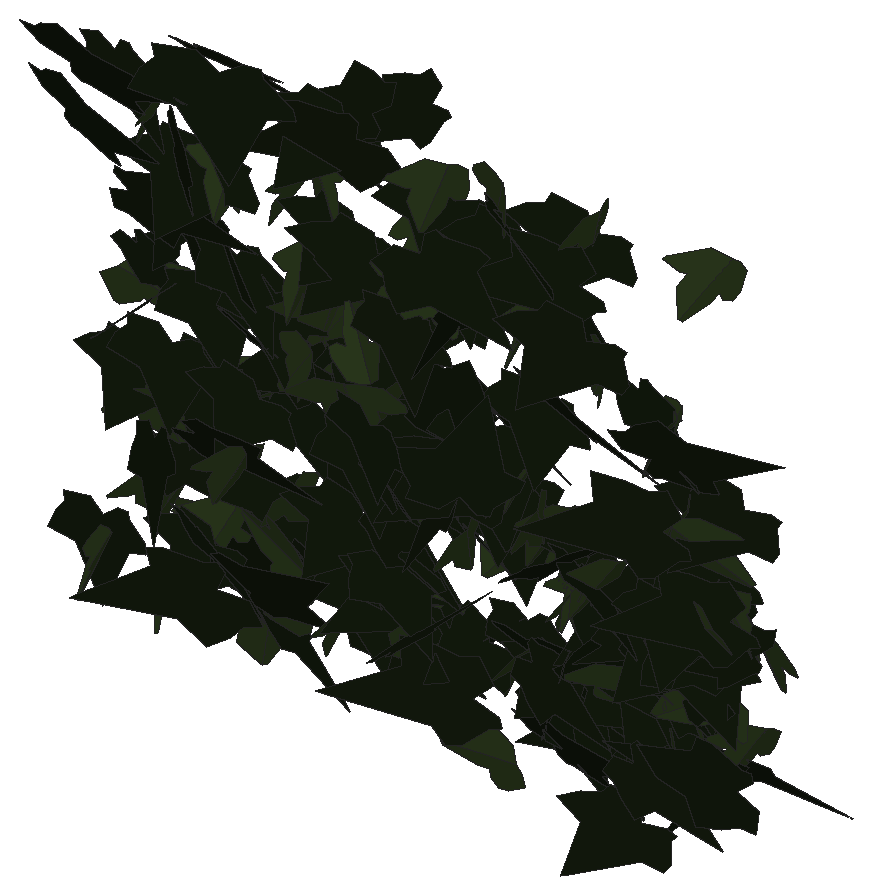
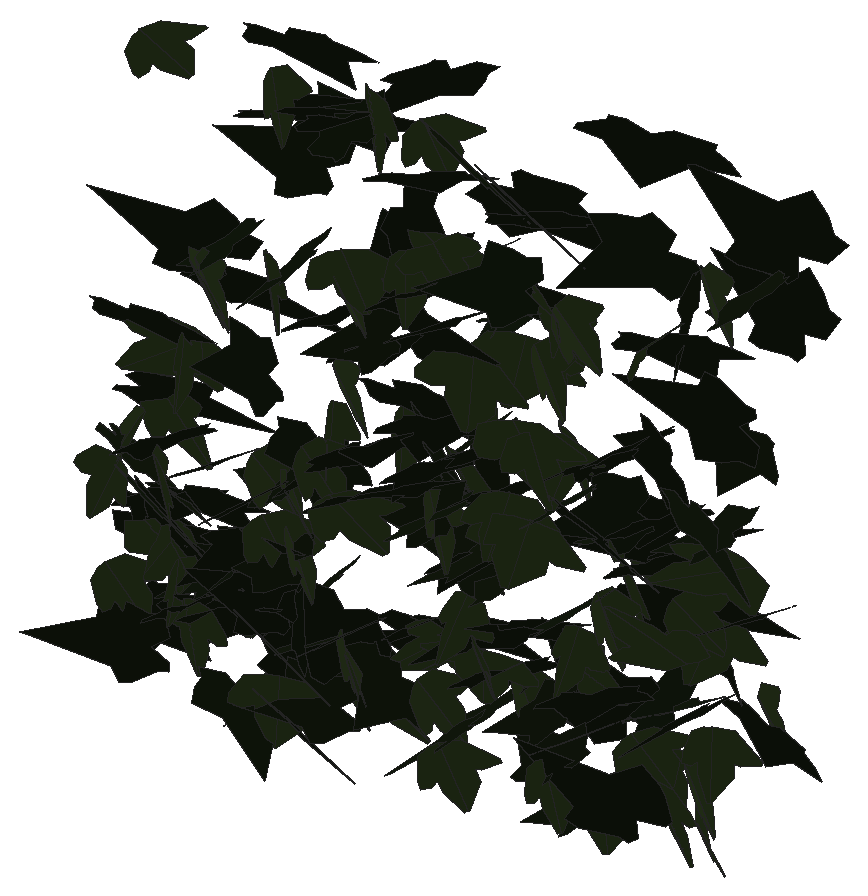
# SketchUp Ruby script. Lengths in millimetres.
U = 1.mm
M = Sketchup.active_model
def pt(a) = Geom::Point3d.new(a.map { |v| v * U })
def face(e, loops, mat)
  f = e.add_face(loops[0].map { |a| pt(a) })
  loops[1..].each { |l| e.add_face(l.map { |a| pt(a) }).erase! }
  f.material = f.back_material = mat if mat
  f
end
# faces: each face lists its corners as indices into pts; further lists are holes
def faces(e, pts, list, mat = nil) = list.each { |f| face(e, (f[0].is_a?(Array) ? f : [f]).map { |l| l.map { |i| pts[i] } }, mat) }
# xy, xz, yz: faces in a plane at the given z, y or x. An outline is a flat list of corners, or four numbers for a rectangle; further outlines are holes
def ring(l) = l.size == 4 ? [[l[0], l[1]], [l[2], l[1]], [l[2], l[3]], [l[0], l[3]]] : l.each_slice(2).to_a
def flat(e, list, mat, &to3) = list.each { |f| face(e, (f[0].is_a?(Array) ? f : [f]).map { |l| ring(l).map { |u, v| to3.(u, v) } }, mat) }
def xy(e, z, list, mat = nil) = flat(e, list, mat) { |x, y| [x, y, z] }
def xz(e, y, list, mat = nil) = flat(e, list, mat) { |x, z| [x, y, z] }
def yz(e, x, list, mat = nil) = flat(e, list, mat) { |y, z| [x, y, z] }
def lines(e, pts, list) = list.each { |a, b| e.add_line(pt(pts[a]), pt(pts[b])) }
# prism: a flat outline (further loops are holes) pulled along v
def prism(e, loops, v, mat = nil)
  f = face(e, loops, mat); d = Geom::Vector3d.new(v.map { |x| x * U })
  f.pushpull(f.normal.samedirection?(d) ? d.length : -d.length)
end
def box(e, o, s, mat = nil) = prism(e, [[o, [o[0] + s[0], o[1], o[2]], [o[0] + s[0], o[1] + s[1], o[2]], [o[0], o[1] + s[1], o[2]]]], [0, 0, s[2]], mat)
def at(x, y, z, deg = 0) = Geom::Transformation.translation(pt([x, y, z])) * Geom::Transformation.rotation(ORIGIN, Z_AXIS, deg.degrees)
def axes(o, x, y, z) = Geom::Transformation.new([*x, 0, *y, 0, *z, 0, *pt(o).to_a, 1])
def part(name) = M.definitions.add(name)
# library, detail: a bought-in or finely detailed component or shape, given as its bounding box
def library(name, o, s) = part(name).tap { |d| box(d.entities, o, s) }
def detail(e, o, s) = box(e.add_group.entities, o, s)
def put(e, d, t, mat = nil) = e.add_instance(d, t).tap { |i| i.material = mat if mat }
def group(e, t, mat = nil) = e.add_group.tap { |g| g.transformation = t; g.material = mat if mat }.entities
root = M.entities
M.materials.add("efeu1").color = [18, 25, 13]
M.materials.add("efeu2").color = [43, 57, 29]
c1 = part("ivyleaf_9")
p = [[39.1,54.8,31.7],[34.5,51.8,30.2],[-5.3,25.2,17.3],[-17.9,28.3,20.9],[-21.6,21.7,17],[-20.2,4.3,5.3],
  [-22.9,-0.3,2.5],[-17.1,-4,-0.6],[-2,-2.1,-1.2],[-0.7,-15.4,-10.1],[16.6,-22.3,-16.7],[21.1,-15.1,-12.5],
  [32.7,-10.7,-11],[46.1,-1.8,-6.6],[30.8,11.2,3.8]]
faces(c1.entities,p,[[0,1,2,3,4,5,6,7,8,9,10,11,12,13,14]],"efeu1")
c2 = part("ivyleaf_10")
p = [[0,12.8,-0.8],[-1.5,51.3,-10.9],[-4.9,51,-11.6],[-13.6,26.5,-7.3],[-13.2,15.9,-4.6],[-21.1,19.3,-7.2],
  [-29.5,16.3,-8.3],[-29.2,8.3,-6.2],[-19.7,-9.8,0.5],[-7.6,-13,4],[1,-12.2,5.8],[-0.4,51.1,-11.1],
  [-1.5,51.1,-10.9],[1,-12.4,5.9],[16.9,-12.4,3.5],[35.1,9.1,-5.1],[35,12.9,-6.1],[20.5,16.4,-4.9],
  [15.8,15,-3.8],[15.3,27.6,-7.1],[12.8,31.3,-7.8]]
faces(c2.entities,p,[[0,1,2,3,4,5,6,7,8,9,10],[11,12,0,13,14,15,16,17,18,19,20]],"efeu2")
put(root,c1,axes([4484.2,737.5,3875.5],[-0.8662,1.10166,0.24911],[-0.165,0.23371,-1.19194],[-2.14327,-0.46323,-0.00892]))
put(root,c1,axes([4459.5,709.3,3735.8],[-0.96321,-0.9947,0.53894],[-0.20052,-0.5464,-1.10741],[2.14378,-0.49803,0.13856]))
put(root,c2,axes([4467.5,721.5,3596.6],[-0.86364,-1.04343,-0.31555],[0.17824,0.30321,-1.13733],[2.067,-0.46211,-0.03377]))
put(root,c2,axes([4468,752.7,3565.3],[0.53503,-1.1435,-0.00813],[-0.00022,0.00834,-1.17754],[2.17636,0.28112,0.00188]))
put(root,c2,axes([4435.2,734,3821.6],[-1.37809,-0.18698,-0.966],[1.82849,0.12448,-0.74424],[0.40412,-1.20082,0.07327]))
put(root,c1,axes([4461.7,639.2,3582.3],[-1.55529,-0.09349,-0.84368],[1.60644,0.03448,-0.8214],[0.17102,-1.17406,0.04306]))
put(root,c1,axes([4428.3,626.2,4066],[0.57945,-0.52323,1.26611],[1.26844,-1.07659,-0.60518],[2.27796,0.73257,0.01492]))
put(root,c1,axes([4449,679.6,4116.3],[0.58104,-1.2282,0.10539],[0.03307,-0.10428,-1.26555],[2.34587,0.30568,-0.00826]))
put(root,c1,axes([4443.8,727.2,3860.5],[1.19269,-1.05488,-0.11701],[0.07243,0.15814,-1.22177],[2.01866,0.61758,0.11298]))
put(root,c2,axes([4489,602.3,3576.7],[0.91486,-1.10236,0.33779],[0.23284,-0.31513,-1.20254],[2.18191,0.49584,-0.01331]))
put(root,c2,axes([4488,697,3710.9],[-1.52452,-0.79664,-0.36954],[0.60599,0.20268,-1.12711],[1.55762,-0.85857,0.07681]))
put(root,c2,axes([4478.8,723.8,3487.3],[1.07034,-0.82353,0.69398],[0.78048,-0.56017,-0.99706],[1.89522,0.69578,0.01867]))
put(root,c2,axes([4505.4,756.8,3531.8],[1.26727,-0.76445,-0.64907],[-0.6013,0.57953,-1.00667],[1.8114,0.72719,0.11993]))
put(root,c2,axes([4504.1,722.3,3742.3],[-0.3921,-0.98037,0.64481],[-0.09794,-0.64649,-0.99937],[2.23109,-0.20068,0.06945]))
put(root,c1,axes([4474.9,732,3640],[1.01558,-0.82192,-0.80551],[-0.3437,0.81709,-0.95336],[2.16312,0.51572,0.22671]))
put(root,c1,axes([4454.8,603.3,4140.8],[0.36317,-0.55782,1.32464],[1.90614,-0.90682,-0.52615],[1.962,0.98426,0.26598]))
put(root,c2,axes([4520,660,4100.1],[0.53963,-1.20234,0.01427],[0.00167,-0.01445,-1.23532],[2.28845,0.28353,-0.00246]))
put(root,c1,axes([4475,678.5,3958.7],[1.14375,0.01997,-1.10127],[1.97965,0.40232,0.57492],[0.68946,-1.18831,0.17613]))
put(root,c1,axes([4514.8,660.5,3681.5],[-1.14316,0.20524,-1.24958],[2.20985,-0.46265,-0.63412],[-0.96176,-1.30698,0.02824]))
put(root,c2,axes([4501.1,750.7,3705.5],[1.49383,0.28257,-0.86056],[1.54485,0.28582,0.83421],[0.76489,-1.12913,-0.00419]))
put(root,c1,axes([4542.6,571.9,3879.2],[0.52058,0.98132,0.76722],[0.40074,0.73777,-1.01872],[-2.33658,0.34517,-0.00378]))
put(root,c1,axes([4527.6,672.3,3796.7],[-0.61984,-1.20389,0.10958],[-0.00016,-0.11346,-1.24681],[2.30071,-0.32435,0.02944]))
put(root,c2,axes([4549.4,740.6,3572.4],[-0.91882,-0.92583,0.60935],[0.08412,-0.6802,-0.99846],[2.10776,-0.37644,0.30548]))
put(root,c2,axes([4550.2,698.7,3524.4],[0.09682,-1.07595,0.45158],[0.32933,-0.44006,-1.06799],[2.19624,0.11342,0.14024]))
put(root,c1,axes([4539.4,724.4,3841.2],[-0.323,-1.21507,-0.17882],[0.00039,0.18049,-1.22662],[2.33742,-0.16794,-0.02451]))
put(root,c1,axes([4568,680.4,4027.5],[-1.88136,-0.81503,-0.06027],[0.0859,0.04,-1.28119],[1.55302,-0.98955,-0.00215]))
put(root,c1,axes([4571.8,625,4072.8],[1.01088,-0.29829,-1.28915],[-2.04316,0.71496,-0.60774],[1.47225,1.19702,0.04175]))
put(root,c1,axes([4526.6,725.2,3913.5],[0.11109,-0.28146,-1.20012],[2.31519,-0.18103,0.10162],[-0.37917,-1.18782,0.26888]))
put(root,c1,axes([4571.3,701.3,3768.2],[-1.01105,-1.08065,0.28391],[-0.196,-0.26567,-1.20392],[2.11743,-0.54059,0.02412]))
put(root,c1,axes([4536.5,774.6,3508.1],[0.1713,-0.19273,1.21554],[2.1972,-0.40909,-0.15035],[0.81161,1.14816,0.15047]))
put(root,c1,axes([4580.7,676.1,3573],[-1.10301,-0.86263,0.60045],[-0.11905,-0.65616,-1.00304],[1.99677,-0.51564,0.27188]))
put(root,c1,axes([4554.6,698.8,4147.1],[2.34527,-0.00824,0.08599],[0.16308,0.27253,-1.20181],[-0.02086,1.20484,0.27243]))
put(root,c2,axes([4593.8,745.3,3724.4],[-0.00027,-1.20744,0.01009],[-0.00059,-0.01009,-1.20744],[2.29809,-0.00014,-0.00031]))
put(root,c2,axes([4580,697.9,4015.7],[-0.75057,-0.50394,1.0881],[1.04138,-1.09486,-0.30875],[2.03074,0.37519,0.5605]))
put(root,c1,axes([4565,673.5,3586.4],[1.01924,-1.02212,0.40608],[0.29613,-0.37671,-1.15339],[2.07214,0.55659,-0.03491]))
put(root,c2,axes([4609.8,684.8,3724.1],[1.09141,-1.06817,-0.28581],[-0.1145,0.29134,-1.20956],[2.10134,0.57067,0.08254]))
put(root,c1,axes([4589.4,707,3906.1],[0.10474,-1.22935,-0.15101],[-0.02573,0.15056,-1.23056],[2.35714,0.05627,-0.00672]))
put(root,c2,axes([4621.5,717.6,3480.9],[-1.48372,-0.93319,-0.00787],[0.02499,-0.00072,-1.21594],[1.77594,-0.77963,0.01054]))
put(root,c1,axes([4605.4,755.6,3620.9],[-0.66255,-1.09279,-0.28599],[0.13502,0.27752,-1.14678],[2.14559,-0.35491,-0.01615]))
put(root,c1,axes([4587.8,708.3,3827.4],[1.96059,-0.62215,0.06083],[0.10631,-0.02518,-1.20343],[1.18496,1.03164,0.00732]))
put(root,c2,axes([4640.3,782.5,3524.9],[-0.60416,-1.10789,-0.0389],[0.00547,0.03964,-1.15245],[2.10983,-0.31735,-0.00815]))
put(root,c1,axes([4621.2,763.6,3567.5],[-0.42067,-1.12341,0.28174],[0.02195,-0.28894,-1.1431],[2.20419,-0.21153,0.06515]))
put(root,c1,axes([4636.7,678.5,3766.8],[-1.15837,-0.84756,0.59812],[-0.06479,-0.67677,-0.99367],[1.97323,-0.51978,0.31849]))
put(root,c1,axes([4616.6,762.1,3722.4],[0.4707,-1.16077,-0.07889],[-0.01074,0.07946,-1.18678],[2.21425,0.24714,0.01101]))
put(root,c1,axes([4673.5,720.4,3805.5],[-2.05586,0.53868,0.08199],[-0.15178,0.0238,-1.20699],[-1.02586,-1.08306,0.01426]))
put(root,c1,axes([4633,715.9,3872.8],[-0.44541,-1.20485,0.00017],[-0.00078,-0.0001,-1.22737],[2.29307,-0.23403,-0.00039]))
put(root,c1,axes([4621.4,734.5,3478.8],[1.26235,-1.02238,-0.06829],[-0.05804,0.06162,-1.21866],[1.94927,0.66393,0.00794]))
put(root,c2,axes([4684.5,674.4,3592.9],[-0.12017,0.0881,-1.26129],[-1.48621,0.99049,0.10827],[1.89252,0.78343,0.00494]))
put(root,c1,axes([4692.5,533.6,3623.1],[-0.30289,-0.22662,-1.32348],[-1.09612,-1.19241,0.27343],[-2.3085,0.59591,0.04382]))
put(root,c1,axes([4616.8,611.3,3746.2],[2.07647,-0.14552,0.48254],[0.89786,-0.11007,-1.09987],[0.33757,1.1879,-0.0428]))
put(root,c2,axes([4658.2,712.4,3647.2],[-0.436,-0.9441,-0.70391],[0.42852,0.66876,-0.97023],[2.19991,-0.31738,0.04948]))
put(root,c2,axes([4668.5,611.9,3740.9],[-0.47289,-1.19559,0.25512],[-0.06745,-0.25318,-1.22103],[2.3257,-0.25044,0.01646]))
put(root,c2,axes([4669.3,714.9,4031.6],[0.10812,-1.18756,0.38494],[-0.05977,-0.38657,-1.18797],[2.37517,0.04433,-0.04742]))
put(root,c1,axes([4641.2,772.2,3532.7],[0.16126,-0.87773,0.74277],[0.57752,-0.70131,-0.86335],[2.11078,0.25894,0.17947]))
put(root,c1,axes([4658.3,587.7,4202.1],[-1.7288,-0.84881,-0.71897],[1.0138,0.48297,-1.24319],[1.85857,-1.05299,0.00935]))
put(root,c1,axes([4635.7,665.8,3548],[2.33681,0.05822,-0.30725],[0.55801,0.21859,1.2131],[0.20697,-1.24667,0.19835]))
put(root,c2,axes([4692.2,731.4,3876.6],[-1.41806,-0.96458,0.06572],[-0.06163,-0.05802,-1.2188],[1.83901,-0.74573,0.00983]))
put(root,c1,axes([4664.6,738.5,3817.4],[0.1785,-1.20055,0.13025],[0.04287,-0.12888,-1.20415],[2.2979,0.09567,0.01235]))
put(root,c2,axes([4695.2,755.3,3782.9],[-2.13466,-0.3878,-0.16179],[0.271,0.0831,-1.18634],[0.75239,-1.13017,-0.03172]))
put(root,c2,axes([4717.6,736.7,3883.8],[-2.10857,-0.23795,0.45365],[-0.78193,-0.2329,-1.12554],[0.58234,-1.17432,0.13131]))
put(root,c2,axes([4701.6,714.1,3970.7],[0.20914,-1.23376,0.036],[0.00977,-0.03569,-1.23864],[2.34907,0.10999,0.00195]))
put(root,c1,axes([4669.9,732.2,3569.3],[1.39202,-0.91981,-0.06111],[-0.04517,0.05919,-1.17502],[1.75386,0.73157,0.01824]))
put(root,c2,axes([4707.7,663.5,3849.7],[1.12382,-0.97092,-0.40967],[-0.30561,0.38122,-1.13494],[1.98219,0.60925,0.05728]))
put(root,c2,axes([4684.7,728.2,4037.2],[-0.76861,0.31003,-1.11864],[0.6974,-1.0898,-0.43433],[-2.09629,-0.47623,0.26566]))
put(root,c2,axes([4707.3,670.3,3959],[-0.13564,-0.80874,0.97025],[0.78982,-0.93284,-0.74707],[2.2705,0.27619,0.31784]))
put(root,c2,axes([4721.5,751.5,3803.9],[-1.30567,-0.93093,-0.32293],[0.57496,0.17582,-1.14865],[1.78501,-0.73758,0.13377]))
put(root,c1,axes([4737.2,695.3,4124.1],[-1.79141,-0.79553,0.25258],[-0.1631,-0.28657,-1.22195],[1.58013,-0.93148,0.16022]))
put(root,c1,axes([4768,701.1,4147.9],[-1.46445,0.89212,0.46128],[-0.63224,0.32231,-1.1775],[-1.80384,-0.83724,0.03822]))
put(root,c1,axes([4770.5,669.7,4130.9],[-0.03604,0.0737,-1.25395],[-1.58292,-0.94053,-0.04272],[-1.7915,0.82954,0.06297]))
put(root,c1,axes([4740.6,722,3643.5],[-1.54759,-0.82316,0.29498],[-0.18295,-0.31623,-1.14743],[1.65411,-0.80513,0.14908]))
put(root,c2,axes([4750.3,684.8,3550.4],[0.08651,-1.20316,-0.00895],[-0.0033,0.00889,-1.20402],[2.28991,0.04547,-0.00139]))
put(root,c1,axes([4752.6,696.5,4000.3],[-1.38668,-0.83948,0.60918],[-0.15473,-0.69595,-1.05628],[1.96796,-0.64624,0.3462]))
put(root,c1,axes([4738.5,730.5,3695.8],[0.2166,-1.15504,0.28047],[0.13801,-0.27448,-1.1598],[2.25793,0.12758,0.04398]))
put(root,c1,axes([4720.8,730.6,4057.6],[1.81193,-0.71718,0.30665],[0.60199,-0.08732,-1.18621],[1.35693,0.99639,0.11677]))
put(root,c1,axes([4757.8,712.9,3577.8],[-0.4265,-1.20586,-0.16397],[0.04267,0.16261,-1.22648],[2.31572,-0.22509,-0.0076]))
put(root,c2,axes([4779,733.8,3618.3],[0.933,-1.07724,-0.05366],[-0.00156,0.05857,-1.18331],[2.05274,0.48966,0.02349]))
put(root,c2,axes([4775,756.1,3664.7],[-0.40702,-0.89408,-0.81791],[0.48366,0.77898,-0.91798],[2.25492,-0.32847,0.04926]))
put(root,c1,axes([4753.8,730.3,3634.2],[0.45173,-0.79333,-0.84105],[0.27967,0.87233,-0.78136],[2.18258,0.05242,0.27419]))
put(root,c2,axes([4789.2,769.2,3486.6],[-0.93366,-1.02197,0.2909],[-0.03387,-0.31246,-1.12773],[2.022,-0.47713,0.11543]))
put(root,c1,axes([4762.1,715,3850.8],[0.24003,-1.12315,-0.43539],[0.17427,0.44544,-1.12256],[2.28594,0.08398,0.13129]))
put(root,c1,axes([4802.4,666.8,4005.1],[-2.01702,-0.61772,0.08652],[-0.15148,-0.03525,-1.22665],[1.17742,-1.06275,-0.0096]))
put(root,c2,axes([4777.5,719,3588.5],[2.18745,0.31036,0.07747],[0.14171,0.02141,-1.19052],[-0.59207,1.15176,0.00126]))
put(root,c1,axes([4768.3,713.2,3528.9],[0.53736,-1.1379,0.02621],[0.01114,-0.02555,-1.17241],[2.1662,0.28241,-0.00047]))
put(root,c2,axes([4804.6,711.5,3920.3],[-2.32084,-0.01407,0.12592],[-0.24004,0.01907,-1.21935],[0.0229,-1.22578,-0.02042]))
put(root,c1,axes([4789.9,677.6,3768.5],[-0.47047,-1.22327,-0.03463],[0.00642,0.03465,-1.24799],[2.32906,-0.2472,-0.00356]))
put(root,c1,axes([4783.2,747.7,3515.1],[1.25937,-0.69093,-0.69381],[-0.48992,0.68518,-0.92784],[1.79799,0.67065,0.23315]))
put(root,c1,axes([4843.3,706.8,4181.8],[-2.04593,0.5842,-0.24994],[0.32728,-0.20539,-1.21968],[-1.16421,-1.08439,0.09636]))
put(root,c1,axes([4842.9,693.3,3599.8],[-1.99369,-0.44709,0.3561],[-0.6322,-0.12882,-1.13891],[0.88526,-1.09889,-0.01137]))
put(root,c1,axes([4806.4,711.5,3587.5],[0.02012,-1.17001,0.11036],[0.03835,-0.11017,-1.16991],[2.23633,0.01241,0.01907]))
put(root,c2,axes([4831.1,589.6,3883],[-2.07111,-0.53728,-0.16161],[0.26344,0.08466,-1.21354],[1.0348,-1.0969,-0.0145]))
put(root,c2,axes([4842.9,661.6,3863.2],[0.163,-1.18686,0.26369],[-0.01581,-0.26491,-1.18965],[2.31386,0.0818,-0.0267]))
put(root,c2,axes([4846.3,724.9,3524.6],[-0.18224,-1.11654,0.51532],[-0.06504,-0.51427,-1.1206],[2.3395,-0.10127,0.00899]))
put(root,c2,axes([4846.9,592.1,3920.2],[0.01191,1.18118,-0.33334],[-0.08397,0.33335,1.18037],[2.33432,0.00597,0.04416]))
put(root,c1,axes([4815.2,675.2,3681.5],[1.11381,-0.97766,-0.35902],[-0.11823,0.37831,-1.13147],[1.97864,0.57295,0.13449]))
put(root,c1,axes([4807.5,646.3,3775.4],[1.25811,-0.38263,-1.12476],[1.98247,-0.43235,0.75929],[-1.08741,-1.23091,0.08294]))
put(root,c2,axes([4858.2,699.2,3733.1],[0.02971,-1.19293,-0.36658],[-0.06971,0.36602,-1.19264],[2.37414,0.02568,-0.03043]))
put(root,c2,axes([4855.1,702.7,4044.5],[1.11257,0.97134,-0.52329],[-0.67253,-0.39618,-1.13015],[-1.98924,0.6772,0.08942]))
put(root,c1,axes([4835.9,733.3,3808.1],[0.04606,-1.10169,-0.44547],[-0.07023,0.44465,-1.10167],[2.26057,0.03626,-0.02515]))
put(root,c2,axes([4863.2,651.8,3763.8],[1.52713,-0.86614,-0.24766],[-0.28064,0.2009,-1.18037],[1.69138,0.81537,0.02776]))
put(root,c1,axes([4847.4,642.3,3655.6],[-0.00525,-1.11264,-0.44385],[-0.05349,0.44379,-1.11231],[2.27922,0.00785,-0.02713]))
put(root,c1,axes([4844.8,725.7,3734.9],[0.04192,-1.17693,0.31025],[0.16068,-0.30808,-1.17468],[2.31088,0.04277,0.07605]))
put(root,c1,axes([4863.7,714.3,3952.7],[-0.89651,-0.99751,0.48523],[-0.19471,-0.48585,-1.09811],[2.10217,-0.47041,0.10523]))
put(root,c1,axes([4847.7,630.8,3797.6],[1.26106,-0.83511,-0.79781],[-0.56559,0.76553,-1.04814],[2.12409,0.69964,0.19456]))
put(root,c2,axes([4853.3,680.9,3571.1],[-0.87238,-0.53801,-0.98206],[1.31023,0.70151,-0.70564],[1.6808,-0.82609,0.04036]))
put(root,c1,axes([4868.9,756.1,3776],[-1.00263,-1.03663,0.25903],[0.0194,-0.29367,-1.1545],[2.03348,-0.50832,0.13873]))
put(root,c2,axes([4896.5,641.2,4007.7],[1.89817,-0.34559,-0.64031],[-1.17866,0.16712,-1.05484],[0.72694,1.17336,-0.03835]))
put(root,c1,axes([4864.3,725.7,4001.9],[-0.31955,-1.22182,-0.05686],[0.01325,0.05644,-1.23331],[2.32786,-0.16805,-0.00079]))
put(root,c2,axes([4883.1,715.3,4020.5],[-0.53083,-1.12787,-0.34975],[0.19506,0.33489,-1.1617],[2.23891,-0.29659,0.01829]))
put(root,c1,axes([4874.2,681.1,3823.2],[-0.77646,-1.06567,-0.40812],[0.19843,0.3968,-1.14033],[2.16275,-0.419,-0.0419]))
put(root,c1,axes([4883.8,730.3,3532.4],[0.68264,0.84748,0.81551],[0.56299,0.76017,-0.92009],[-2.16645,0.46458,0.01786]))
put(root,c1,axes([4852.5,699.9,3731.6],[1.4288,-0.93582,0.37261],[0.39988,-0.309,-1.1994],[1.87487,0.77907,-0.02814]))
put(root,c1,axes([4942.4,648.2,3531.5],[-2.06192,-0.07843,0.84395],[-1.60303,-0.05332,-1.08621],[0.18012,-1.37228,-0.00603]))
put(root,c1,axes([4882.9,560.8,3872.6],[-0.10473,-1.06245,0.60991],[0.02686,-0.61103,-1.06314],[2.3314,-0.04068,0.03965]))
put(root,c2,axes([4907.2,648.2,4144.3],[-0.91667,-1.05232,0.44016],[0.23083,-0.52233,-1.11605],[2.15861,-0.39102,0.30627]))
put(root,c1,axes([4888.6,609.8,3977.7],[-0.20733,-1.25254,0.23472],[-0.03663,-0.23393,-1.25727],[2.42505,-0.11062,0.00108]))
put(root,c1,axes([4949.7,622.6,3878.9],[-0.26451,0.19601,1.4464],[-1.30749,1.27316,-0.23855],[-2.45102,-0.70032,-0.02884]))
put(root,c1,axes([4915.9,712.7,3559.9],[-0.98735,-0.74615,0.8101],[-0.65056,-0.74218,-0.90248],[1.99261,-0.61203,0.10676]))
put(root,c1,axes([4907.4,668.4,4102.3],[-1.29995,-1.03968,0.03527],[0.26685,-0.13382,-1.22929],[1.9618,-0.67072,0.19059]))
put(root,c2,axes([4917.4,763.9,3545.2],[0.82879,-1.08578,-0.13815],[0.01467,0.15172,-1.16815],[2.08307,0.43093,0.06319]))
put(root,c1,axes([4926.1,635,3773.8],[-1.46458,0.54326,-0.84018],[1.31987,-0.47439,-0.94193],[-1.37253,-1.03588,-0.00926]))
put(root,c1,axes([4909.3,572.2,3612.4],[-0.35656,1.29671,-0.4513],[-0.11792,0.44704,1.31017],[2.61043,0.19731,-0.00246]))
put(root,c1,axes([4958.6,633.5,3809.4],[-2.35034,-0.25607,0.11644],[-0.21751,-0.02234,-1.26121],[0.48919,-1.24022,-0.00133]))
put(root,c2,axes([4979,665,3462.3],[-0.63448,0.2022,1.11857],[-2.11283,0.19256,-0.36567],[-0.46486,-1.1512,0.1353]))
put(root,c2,axes([4948.7,731.6,3547.7],[0.1192,-1.22048,-0.17991],[-0.05092,0.17875,-1.22197],[2.34737,0.06585,-0.01737]))
put(root,c2,axes([4954.3,728.7,4005.1],[-1.60873,-0.81197,0.36804],[0.03176,-0.5215,-1.11221],[1.69639,-0.76025,0.36985]))
put(root,c2,axes([4965.8,723.2,3704.6],[-1.2608,-0.72618,0.68666],[-0.3902,-0.70755,-0.94607],[1.86165,-0.64011,0.26675]))
put(root,c1,axes([4958.7,624.3,4022.6],[-0.60811,0.5689,-1.11645],[1.11713,-0.94999,-0.65207],[-2.10696,-0.6679,-0.0235]))
put(root,c1,axes([4941.5,753.1,3573],[-0.02871,-1.14507,0.06503],[0.02871,-0.06523,-1.14506],[2.18262,-0.01421,0.01592]))
put(root,c1,axes([4949.8,695.4,3773.3],[-0.67287,-1.14373,0.02371],[-0.01436,-0.02248,-1.19712],[2.17716,-0.35363,-0.00057]))
put(root,c1,axes([4951.3,720.2,3723.1],[-0.48685,-1.17212,-0.08039],[0.02237,0.07971,-1.1997],[2.23591,-0.25602,-0.0055]))
put(root,c2,axes([4970.7,608.8,3754],[-0.06725,-1.14369,-0.54348],[0.23359,0.53804,-1.14022],[2.39858,-0.08447,0.09581]))
put(root,c1,axes([4969.2,719.2,3576.5],[1.92833,0.33232,-0.50112],[-0.91883,-0.13571,-1.06613],[-0.68217,1.12218,0.01947]))
put(root,c2,axes([4973.3,712.9,3969.9],[0.8119,-1.13929,0.21512],[0.11652,-0.20676,-1.21645],[2.20354,0.43071,-0.01493]))
put(root,c2,axes([4979.6,649.8,4151.9],[1.34618,-0.94028,-0.41999],[0.05216,0.52652,-1.13262],[1.95924,0.63204,0.31873]))
put(root,c1,axes([4938.2,770,3496.8],[1.88581,-0.36703,0.46081],[1.03473,0.22244,-0.99187],[0.43181,1.0699,0.3643]))
put(root,c1,axes([4952.4,666.1,3893.8],[1.67245,-0.86198,0.0072],[0.02737,0.00437,-1.23088],[1.64036,0.87878,0.01319]))
put(root,c1,axes([4977.7,649.7,3864.3],[-0.75286,-1.15691,0.0657],[-0.03231,-0.06363,-1.22266],[2.20513,-0.39592,0.00452]))
put(root,c1,axes([4969.9,694.9,3761.7],[0.73293,-0.79395,-0.89057],[-0.22002,0.90658,-0.85821],[2.26001,0.34574,0.20527]))
put(root,c1,axes([4964.5,739,3489.2],[1.34839,-0.93862,0.00574],[-0.0018,-0.0079,-1.17598],[1.78641,0.70846,-0.00551]))
put(root,c2,axes([5004.9,781.7,3497.1],[-1.85242,-0.61456,-0.04753],[0.04849,0.04865,-1.15078],[1.17213,-0.97327,-0.02751]))
put(root,c1,axes([5030.7,772.9,3472],[-1.83487,0.6224,0.12997],[-0.20188,0.07532,-1.14753],[-1.19314,-0.9699,-0.00572]))
put(root,c1,axes([5001.9,739,3535.8],[-1.09109,-0.70023,0.75452],[-0.29631,-0.79473,-0.85583],[1.93658,-0.51612,0.29416]))
put(root,c2,axes([5005.8,670.1,3822.5],[0.76314,-1.14063,0.09568],[0.01328,-0.09894,-1.20878],[2.17843,0.40019,-0.02615]))
put(root,c2,axes([5010.7,715.3,3743],[-0.25498,-1.11855,0.43094],[-0.01654,-0.4327,-1.12583],[2.28129,-0.12816,0.04]))
put(root,c2,axes([5020.9,732,3649.3],[0.21029,-1.18793,-0.14228],[-0.0655,0.13967,-1.19287],[2.27608,0.11377,-0.02118]))
put(root,c1,axes([4989.7,517.8,4132.3],[0.36735,-0.92808,-1.03853],[-0.00105,1.0484,-0.937],[2.65076,0.12903,0.14355]))
put(root,c1,axes([5010.1,739.3,3563.6],[-0.63897,0.20957,-1.18902],[1.62375,-0.83205,-0.38755],[-1.62586,-0.91333,0.08024]))
put(root,c2,axes([5019.9,665.7,3769.7],[0.0959,-1.07273,-0.61116],[0.22078,0.61307,-1.06653],[2.33932,-0.01388,0.12571]))
put(root,c1,axes([5046.2,771,3552.5],[-1.86092,0.60106,-0.12432],[0.18175,-0.08201,-1.14759],[-1.15393,-0.98224,0.01974]))
put(root,c1,axes([5027.9,636.4,4112.4],[-1.48497,-0.97691,-0.0115],[0.0151,0.00838,-1.25025],[1.85931,-0.78029,0.00097]))
put(root,c1,axes([5022,675.4,3899],[-0.61992,-1.17556,0.2203],[-0.08241,-0.21659,-1.21975],[2.27479,-0.32821,0.01585]))
put(root,c1,axes([5006.1,735.8,3487.9],[0.66459,-1.13536,0.06954],[0.04957,-0.06474,-1.18783],[2.1643,0.35012,0.00585]))
put(root,c1,axes([5045,659.8,3724.3],[0.36262,1.21252,0.02993],[0.00059,0.03025,-1.22739],[-2.30836,0.19048,0.00439]))
put(root,c1,axes([5013.8,674.5,3582.1],[1.21989,-0.8595,-0.77315],[-0.67221,0.69617,-1.06674],[2.09503,0.72384,0.10792]))
put(root,c2,axes([5041.7,747.2,3662.8],[-0.89342,-1.05431,0.34154],[-0.00443,-0.36998,-1.14529],[2.10922,-0.44736,0.14226]))
put(root,c1,axes([5014.5,718.1,3993.5],[1.28342,-0.87735,-0.67896],[-0.64735,0.59278,-1.10382],[2.0097,0.75123,0.07804]))
put(root,c1,axes([5052.8,783.2,3477.5],[0.22689,1.14054,0.05735],[-0.24061,0.07049,-1.13903],[-2.16006,0.11195,0.1329]))
put(root,c1,axes([5009,654.2,4105.8],[0.08735,-0.86139,0.97001],[0.48705,-0.94553,-0.85176],[2.42044,0.22135,0.13639]))
put(root,c1,axes([5043.2,511,3873.3],[-1.40012,-0.51703,1.10661],[1.80946,0.5686,0.89771],[-1.45938,1.20103,0.05138]))
put(root,c2,axes([5042.8,711.6,3686.4],[1.18282,-1.0098,0.3924],[0.36352,-0.34316,-1.18562],[2.02956,0.64997,-0.01633]))
put(root,c1,axes([5031.2,769.4,3471.9],[0.39354,-1.13343,-0.00739],[-0.05362,0.00237,-1.15182],[2.15653,0.2069,-0.02729]))
put(root,c1,axes([5019.7,747.4,3633.7],[1.48238,-0.74968,0.40969],[0.78044,-0.15829,-1.06926],[1.4264,0.86571,0.15927]))
put(root,c1,axes([5024.4,696.6,3482],[0.04203,-0.4541,1.10739],[1.41646,-0.8622,-0.3684],[1.78395,0.69528,0.26642]))
put(root,c2,axes([5071,710.5,3950.7],[0.9788,-0.9749,-0.54171],[-0.08115,0.5789,-1.08233],[2.12107,0.47203,0.20857]))
put(root,c1,axes([5109,617.3,4098.5],[-1.88845,-0.08441,0.75828],[-1.33491,-0.38861,-0.96109],[0.57141,-1.18682,0.26077]))
put(root,c2,axes([5081.2,707.9,3706],[-0.25156,-1.08736,0.51445],[-0.10322,-0.51163,-1.09534],[2.28706,-0.14269,0.00715]))
put(root,c1,axes([5047.4,723.3,3556.6],[0.11717,-0.05828,1.23131],[2.0331,0.61772,-0.02417],[-1.17069,1.06694,0.08125]))
put(root,c1,axes([5102.5,748.5,3635],[-2.17659,-0.31881,0.16691],[-0.31455,-0.02864,-1.18714],[0.60838,-1.15541,-0.01662]))
put(root,c1,axes([5083.3,678.6,4122.6],[-1.61409,-0.90696,0.2864],[-0.0402,-0.36567,-1.22053],[1.80969,-0.81705,0.22833]))
put(root,c1,axes([5057.9,743.7,3643.2],[0.12714,-0.52458,-1.08541],[0.10792,1.08724,-0.52197],[2.29182,-0.0221,0.08479]))
put(root,c2,axes([5087.8,725.7,3577],[-1.50409,-0.84131,-0.05623],[0.06741,0.04387,-1.15428],[1.60334,-0.79108,-0.00422]))
put(root,c1,axes([5053,702.2,3698.7],[0.69772,-1.08139,0.36484],[0.31099,-0.32952,-1.14089],[2.1497,0.39865,0.04663]))
put(root,c2,axes([5093.5,672.1,4147],[-0.03223,-1.25629,-0.14216],[0.22281,0.14,-1.25118],[2.3959,-0.02992,0.11444]))
put(root,c1,axes([5075.5,746.3,3685.9],[0.07677,-1.20572,0.01202],[-0.02681,-0.0125,-1.2063],[2.29468,0.04019,-0.0145]))
put(root,c1,axes([5085,746.9,3545.8],[-0.21892,-0.99117,-0.6294],[0.3524,0.60919,-0.99318],[2.20663,-0.19562,0.09617]))
put(root,c1,axes([5127.8,753,3554.6],[-1.39715,-0.9033,0.06874],[-0.08725,-0.05132,-1.16398],[1.72193,-0.73553,-0.0032]))
put(root,c1,axes([5101.8,746.1,3595.4],[1.20023,-0.9662,-0.27803],[-0.16079,0.27612,-1.15116],[1.90673,0.63148,0.07794]))
put(root,c2,axes([5137.8,761.3,3535.4],[1.70962,-0.61811,-0.43066],[-0.16315,0.58198,-1.0141],[1.42445,0.80851,0.40073]))
put(root,c1,axes([5125.3,653.8,3780.9],[0.77112,0.16812,1.16004],[1.16432,1.01662,-0.36101],[-1.9029,0.69016,0.2492]))
put(root,c1,axes([5136.9,766.4,3548.3],[-0.45776,-1.13583,0.03593],[-0.00963,-0.03565,-1.16101],[2.16276,-0.24056,0.00243]))
put(root,c2,axes([5151.6,760.6,3578.5],[-0.02634,-1.14695,-0.22001],[0.59181,0.20846,-1.10632],[2.14244,-0.07169,0.3029]))
put(root,c2,axes([5165.2,701.8,3908.3],[0.64394,-1.17623,0.08488],[0.02109,-0.08513,-1.22386],[2.24433,0.33828,-0.01285]))
put(root,c2,axes([5161.4,715.8,3914.9],[1.20593,-1.03128,0.22207],[0.15647,-0.20999,-1.20975],[2.00162,0.63774,-0.03922]))
put(root,c1,axes([5179.6,715.5,3646],[-1.99541,-0.50566,0.05649],[-0.05945,-0.06516,-1.16315],[0.96654,-1.04795,0.04507]))
put(root,c1,axes([5184.5,629.7,3473.3],[-2.13786,-0.29497,-0.01693],[0.02911,0.00843,-1.16137],[0.56157,-1.12339,-0.00427]))
put(root,c1,axes([5141.6,690.2,3945.9],[0.83461,-1.1551,-0.0698],[-0.04892,0.0649,-1.23554],[2.20185,0.43928,-0.00099]))
put(root,c1,axes([5124.8,559.7,3990.7],[1.31408,-0.84039,0.77859],[1.10668,-0.52618,-1.08361],[1.87862,0.89781,0.09373]))
put(root,c1,axes([5167.2,715.1,3679.4],[-0.68466,-1.08939,0.37573],[-0.04993,-0.38577,-1.14361],[2.19261,-0.34896,0.09128]))
put(root,c1,axes([5223.9,613.8,3845],[-2.17835,0.06612,0.67883],[-1.29407,-0.00656,-1.1458],[-0.10185,-1.33072,0.03938]))
put(root,c2,axes([5179.3,760.7,3694.1],[0.89072,-1.07376,0.00249],[0.24191,0.05271,-1.16321],[2.02922,0.46504,0.13758]))
put(root,c2,axes([5181.3,690.4,3528.4],[0.49135,-0.97901,-0.59637],[0.26689,0.63368,-0.97957],[2.16535,0.14405,0.25606]))
put(root,c1,axes([5169.8,727.4,3577.7],[-1.17684,0.80711,0.73771],[0.72116,-0.63682,1.01434],[1.95212,0.72183,0.07001]))
put(root,c1,axes([5198.7,521.7,4102.7],[-2.17397,-0.52996,-0.07898],[0.13927,0.02994,-1.25922],[1.0102,-1.14461,0.00363]))
put(root,c2,axes([5186.9,707.7,3811.3],[0.03062,-1.06662,-0.66344],[0.25345,0.66121,-1.0598],[2.37717,-0.05676,0.12154]))
put(root,c2,axes([5207.1,725.8,3591],[1.80408,0.02402,-0.71315],[-1.33296,0.25815,-0.92225],[0.25978,1.1578,0.22042]))
put(root,c1,axes([5222.7,757.7,3664.9],[-1.81065,0.70352,-0.09598],[0.15901,-0.04843,-1.18319],[-1.34195,-0.95497,-0.0107]))
put(root,c2,axes([5175.6,750.4,3592.2],[1.15862,-0.84993,0.577],[1.30225,-0.1648,-0.96466],[1.45831,0.82242,0.40301]))
put(root,c1,axes([5184.2,748.4,3724.9],[-0.27776,-1.18109,-0.17242],[0.11588,0.16611,-1.18941],[2.26872,-0.15309,0.03964]))
put(root,c1,axes([5179.5,636.9,3536.5],[1.03658,-0.90417,-0.67064],[-0.1741,0.707,-1.02748],[2.13541,0.49655,0.24178]))
put(root,c2,axes([5243.9,670.3,3710.2],[-1.24001,0.23488,0.97689],[-1.78222,0.27996,-0.69187],[-0.69295,-1.14036,0.03135]))
put(root,c1,axes([5194.5,718,3637.5],[-0.48209,-1.02103,-0.58523],[0.257,0.56946,-1.05197],[2.225,-0.287,-0.00529]))
put(root,c1,axes([5220.8,726.3,3500.7],[-0.59466,0.53168,-1.01304],[0.78575,-0.92699,-0.61385],[-2.03071,-0.51438,0.05914]))
put(root,c1,axes([5264.7,675.8,3724.2],[-1.95539,-0.18444,0.70049],[-1.31812,-0.10601,-1.04374],[0.40387,-1.23897,-0.01497]))
put(root,c2,axes([5202.9,685.8,3803.8],[-1.76632,-0.1007,-0.77885],[1.46432,0.12508,-0.93299],[0.29958,-1.20511,-0.03175]))
put(root,c1,axes([5186.6,777.4,3486.7],[1.81264,-0.36758,0.55902],[1.12704,0.01058,-1.00196],[0.59256,1.1043,0.19567]))
put(root,c2,axes([5242.3,756.7,3541.6],[-0.59389,-1.025,0.45467],[-0.12225,-0.45483,-1.06945],[2.13059,-0.31181,0.06537]))
put(root,c1,axes([5192.4,653.3,3902.7],[0.40826,-0.10207,1.20924],[2.25071,-0.25797,-0.23156],[0.51826,1.20072,0.05304]))
put(root,c1,axes([5255.3,713.7,3835.8],[-2.24936,-0.31478,-0.11874],[0.24644,-0.0253,-1.22173],[0.59097,-1.18756,0.0575]))
put(root,c1,axes([5275.3,707.1,3671.9],[-1.43815,0.88999,0.03043],[-0.28905,-0.08948,-1.15453],[-1.66998,-0.75095,0.17363]))
put(root,c1,axes([5298,646,3546.4],[-1.10747,-0.01429,-1.14079],[-1.99721,-0.49574,0.5415],[-0.85191,1.18078,0.21353]))
put(root,c2,axes([5248.8,718.3,3706.7],[-0.77235,1.06458,0.32695],[-0.20496,0.30883,-1.13927],[-2.10958,-0.41977,-0.00901]))
put(root,c2,axes([5258,675.6,4143.8],[-0.86707,-0.84555,0.79662],[0.02447,-0.85931,-0.90473],[2.21082,-0.32211,0.32245]))
put(root,c2,axes([5253.4,755.1,3665.8],[-1.6177,0.81382,0.03331],[-0.03712,0.02779,-1.17675],[-1.54972,-0.85019,-0.00658]))
